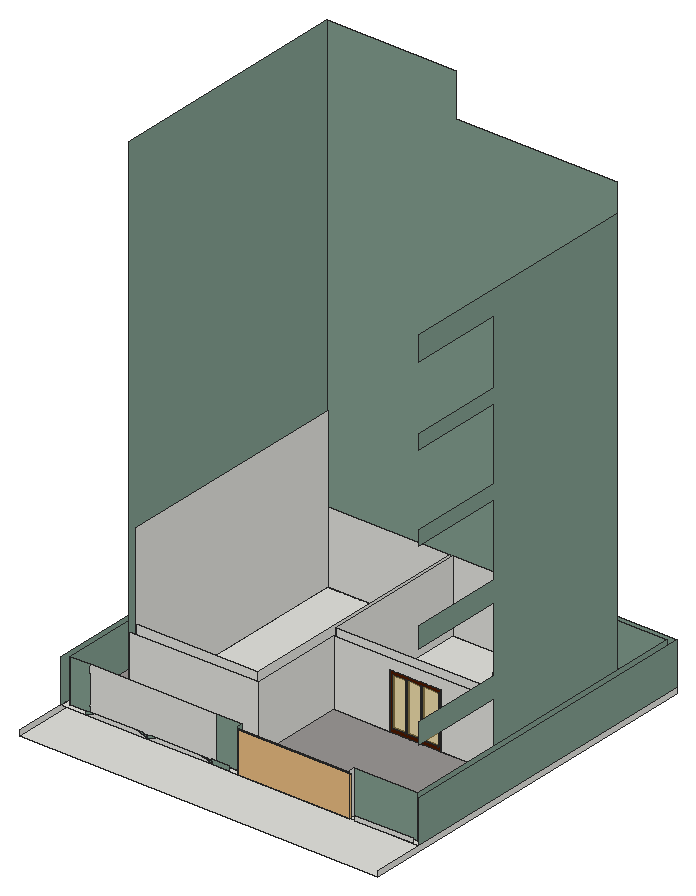
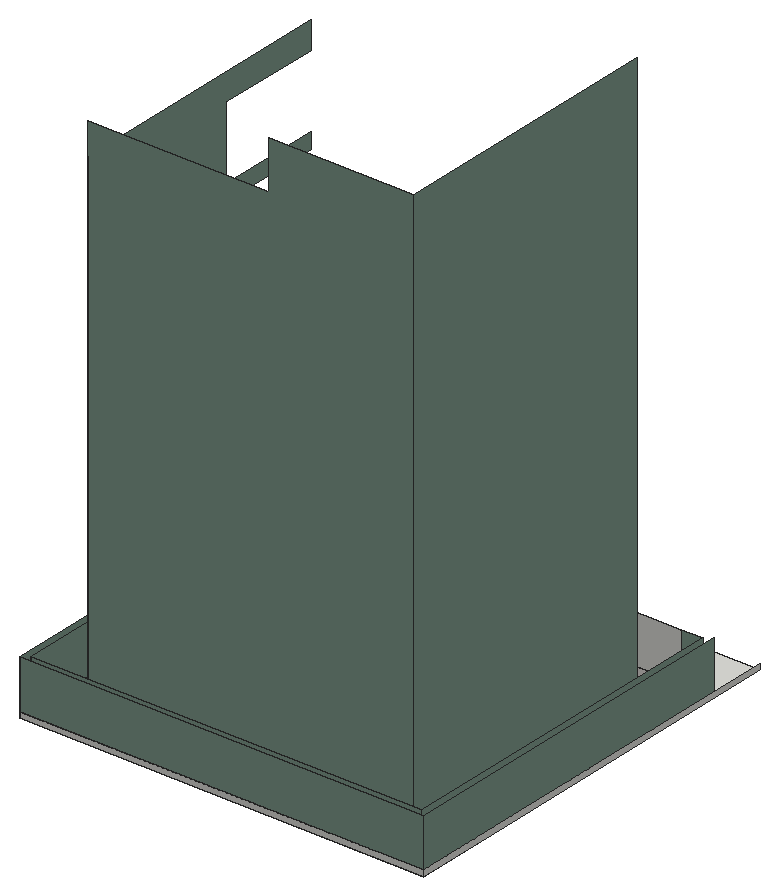
# SketchUp Ruby script. Lengths in inches.
U = 1.inch
M = Sketchup.active_model
def pt(a) = Geom::Point3d.new(a.map { |v| v * U })
def face(e, loops, mat)
  f = e.add_face(loops[0].map { |a| pt(a) })
  loops[1..].each { |l| e.add_face(l.map { |a| pt(a) }).erase! }
  f.material = f.back_material = mat if mat
  f
end
# faces: each face lists its corners as indices into pts; further lists are holes
def faces(e, pts, list, mat = nil) = list.each { |f| face(e, (f[0].is_a?(Array) ? f : [f]).map { |l| l.map { |i| pts[i] } }, mat) }
# xy, xz, yz: faces in a plane at the given z, y or x. An outline is a flat list of corners, or four numbers for a rectangle; further outlines are holes
def ring(l) = l.size == 4 ? [[l[0], l[1]], [l[2], l[1]], [l[2], l[3]], [l[0], l[3]]] : l.each_slice(2).to_a
def flat(e, list, mat, &to3) = list.each { |f| face(e, (f[0].is_a?(Array) ? f : [f]).map { |l| ring(l).map { |u, v| to3.(u, v) } }, mat) }
def xy(e, z, list, mat = nil) = flat(e, list, mat) { |x, y| [x, y, z] }
def xz(e, y, list, mat = nil) = flat(e, list, mat) { |x, z| [x, y, z] }
def yz(e, x, list, mat = nil) = flat(e, list, mat) { |y, z| [x, y, z] }
def lines(e, pts, list) = list.each { |a, b| e.add_line(pt(pts[a]), pt(pts[b])) }
# prism: a flat outline (further loops are holes) pulled along v
def prism(e, loops, v, mat = nil)
  f = face(e, loops, mat); d = Geom::Vector3d.new(v.map { |x| x * U })
  f.pushpull(f.normal.samedirection?(d) ? d.length : -d.length)
end
def box(e, o, s, mat = nil) = prism(e, [[o, [o[0] + s[0], o[1], o[2]], [o[0] + s[0], o[1] + s[1], o[2]], [o[0], o[1] + s[1], o[2]]]], [0, 0, s[2]], mat)
def at(x, y, z, deg = 0) = Geom::Transformation.translation(pt([x, y, z])) * Geom::Transformation.rotation(ORIGIN, Z_AXIS, deg.degrees)
def axes(o, x, y, z) = Geom::Transformation.new([*x, 0, *y, 0, *z, 0, *pt(o).to_a, 1])
def part(name) = M.definitions.add(name)
# library, detail: a bought-in or finely detailed component or shape, given as its bounding box
def library(name, o, s) = part(name).tap { |d| box(d.entities, o, s) }
def detail(e, o, s) = box(e.add_group.entities, o, s)
def put(e, d, t, mat = nil) = e.add_instance(d, t).tap { |i| i.material = mat if mat }
def group(e, t, mat = nil) = e.add_group.tap { |g| g.transformation = t; g.material = mat if mat }.entities
root = M.entities
M.materials.add("[Color B08]1").color = [78, 25, 0]
M.materials.add("[Color H08]").color = [130, 158, 143]
M.materials.add("[Concrete Aggregate Smoke]").color = [154, 150, 148]
M.materials.add("[Translucent Glass Blue]1").color = [221, 188, 93]
M.materials["[Translucent Glass Blue]1"].alpha = 0.5
c1 = library("Group\#4",[0,0,0],[190.73,6,117.875])
xy(root,0,[[0,0,600,625.1875]])
xy(root,9,[[0,85.1875,0,625.1875,600,625.1875,600,85.1875,484.36,85.1875,484.36,94.1875,591,94.1875,591,616.1875,9,616.1875,9,94.1875,42.01,94.1875,42.01,85.1875],[42.01,85.1875,253.1,94.1875],[253.1,85.1875,296.4375,94.1875],[[69,142.1875,69,556.1875,554.1875,556.1875,554.1875,299.125,465.83,299.125,465.83,305.125,548.75,305.125,548.75,550.1875,285.75,550.1875,285.75,305.125,380.7,305.125,380.7,299.125,285.75,299.125,285.75,142.1875],[75,148.1875,279.75,550.1875]],[75,148.1875,279.75,550.1875],
  [285.75,305.125,548.75,550.1875]])
xy(root,9,[[[9,94.1875,591,616.1875],[69,142.1875,69,556.1875,554.1875,556.1875,554.1875,299.125,465.83,299.125,465.83,305.125,380.7,305.125,380.7,299.125,285.75,299.125,285.75,142.1875]]],"[Concrete Aggregate Smoke]")
xz(root,85.1875,[[42.01,9,57.43,16.375,127.49,16.375,144.11,9],[144.11,9,161.86,16.375,236.65,16.375,253.1,9],[493.5625,9,590.375,16.375]])
xz(root,85.1875,[[42.01,9,42.01,12.82,49.44,16.375,57.43,16.375],[144.11,9,144.11,12.91,143.93,12.83,135.91,16.375,127.49,16.375],[144.11,9,144.11,12.91,152.53,16.375,161.86,16.375],[253.1,9,253.1,12.82,245.17,16.375,236.65,16.375],[253.1,9,281.76,16.375]],"[Color H08]")
xz(root,94.1875,[[42.01,9,253.1,81]])
xz(root,94.1875,[[9,9,42.01,81],[253.1,9,296.4375,81],[484.36,9,591,81]],"[Color H08]")
xz(root,142.1875,[[69,9,285.75,118.4375]])
xz(root,148.1875,[[75,9,279.75,129]])
xz(root,299.125,[[285.75,9,380.7,9,380.7,101.5625,465.83,101.5625,465.83,9,554.1875,9,554.1875,118.4375,285.75,118.4375]])
xz(root,305.125,[[285.75,9,285.75,129,548.75,129,548.75,9,465.83,9,465.83,101.5625,380.7,101.5625,380.7,9]])
xz(root,550.1875,[[75,9,279.75,129],[285.75,9,548.75,129]])
xz(root,556.1875,[[69,9,69,853.5,285.75,853.5,285.75,781.5,554.1875,781.5,554.1875,9]],"[Color H08]")
xz(root,616.1875,[[9,9,591,81]],"[Color H08]")
xz(root,625.1875,[[0,0,600,9]])
xz(root,625.1875,[[0,9,600,81]],"[Color H08]")
yz(root,0,[[0,0,625.1875,9]])
yz(root,0,[[85.1875,9,625.1875,81]],"[Color H08]")
yz(root,9,[[94.1875,9,616.1875,81]],"[Color H08]")
yz(root,69,[[142.1875,9,556.1875,853.5]],"[Color H08]")
yz(root,75,[[148.1875,9,550.1875,273]])
yz(root,279.75,[[148.1875,9,550.1875,129]])
yz(root,285.75,[[142.1875,9,299.125,118.4375],[305.125,9,550.1875,129]])
yz(root,296.4375,[[85.1875,9,94.1875,81]],"[Color H08]")
yz(root,380.7,[[299.125,9,305.125,101.5625]])
yz(root,465.83,[[299.125,9,305.125,101.5625]])
yz(root,484.36,[[85.1875,9,94.1875,81]])
yz(root,548.75,[[305.125,9,550.1875,153]])
yz(root,554.1875,[[299.125,9,556.1875,9,556.1875,733.5,142.1875,733.5,142.1875,693.3125,299.125,693.3125,299.125,585,142.1875,585,142.1875,561,299.125,561,299.125,441,142.1875,441,142.1875,417,299.125,417,299.125,297,142.1875,297,142.1875,262.5625,299.125,262.5625,299.125,153,142.1875,153,142.1875,118.4375,299.125,118.4375]],"[Color H08]")
yz(root,591,[[94.1875,9,616.1875,81]],"[Color H08]")
yz(root,600,[[0,0,625.1875,9]])
yz(root,600,[[85.1875,9,625.1875,81]],"[Color H08]")
put(root,c1,axes([296.4375,85.1875,9],[0.98532,0,0],[0,0.5,0],[0,0,0.565]))
g1 = group(root,at(380.7,299.125,9))
xy(g1,0,[[0,0,85.125,0.875],[0,0.875,85.125,3.375]],"[Color B08]1")
xy(g1,5.5,[[3.91,0,27.19,0.875],[29.3,0,52.15,0.875],[54.25,0,81.21,0.875],[3.91,0.875,27.19,3.375],[29.3,0.875,52.15,3.375],
  [54.25,0.875,81.21,3.375]],"[Color B08]1")
xy(g1,87.0625,[[3.91,0,27.19,0.875],[29.3,0,52.15,0.875],[54.25,0,81.21,0.875],[3.91,0.875,27.19,3.375],[29.3,0.875,52.15,3.375],
  [54.25,0.875,81.21,3.375]],"[Color B08]1")
xy(g1,92.5625,[[0,0,85.125,0.875],[0,0.875,85.125,3.375]],"[Color B08]1")
xz(g1,0,[[[0,0,85.125,92.5625],[54.25,5.5,81.21,87.0625],[3.91,5.5,27.19,87.0625],[29.3,5.5,52.15,87.0625]]],"[Color B08]1")
xz(g1,0.875,[[[0,0,85.125,92.5625],[54.25,5.5,81.21,87.0625],[3.91,5.5,27.19,87.0625],[29.3,5.5,52.15,87.0625]]])
xz(g1,0.875,[[3.91,5.5,27.19,87.0625],[29.3,5.5,52.15,87.0625],[54.25,5.5,81.21,87.0625]],"[Translucent Glass Blue]1")
xz(g1,3.375,[[[0,0,85.125,92.5625],[54.25,5.5,81.21,87.0625],[3.91,5.5,27.19,87.0625],[29.3,5.5,52.15,87.0625]]],"[Color B08]1")
yz(g1,0,[[0,0,0.875,92.5625],[0.875,0,3.375,92.5625]],"[Color B08]1")
yz(g1,3.91,[[0,5.5,0.875,87.0625],[0.875,5.5,3.375,87.0625]],"[Color B08]1")
yz(g1,27.19,[[0,5.5,0.875,87.0625],[0.875,5.5,3.375,87.0625]],"[Color B08]1")
yz(g1,29.3,[[0,5.5,0.875,87.0625],[0.875,5.5,3.375,87.0625]],"[Color B08]1")
yz(g1,52.15,[[0,5.5,0.875,87.0625],[0.875,5.5,3.375,87.0625]],"[Color B08]1")
yz(g1,54.25,[[0,5.5,0.875,87.0625],[0.875,5.5,3.375,87.0625]],"[Color B08]1")
yz(g1,81.21,[[0,5.5,0.875,87.0625],[0.875,5.5,3.375,87.0625]],"[Color B08]1")
yz(g1,85.125,[[0,0,0.875,92.5625],[0.875,0,3.375,92.5625]],"[Color B08]1")
